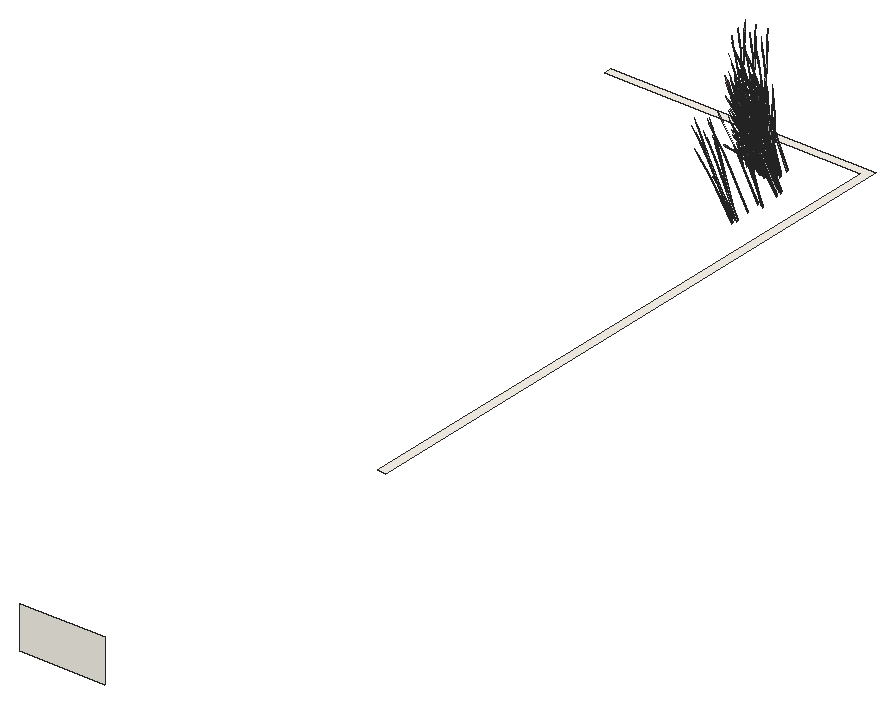
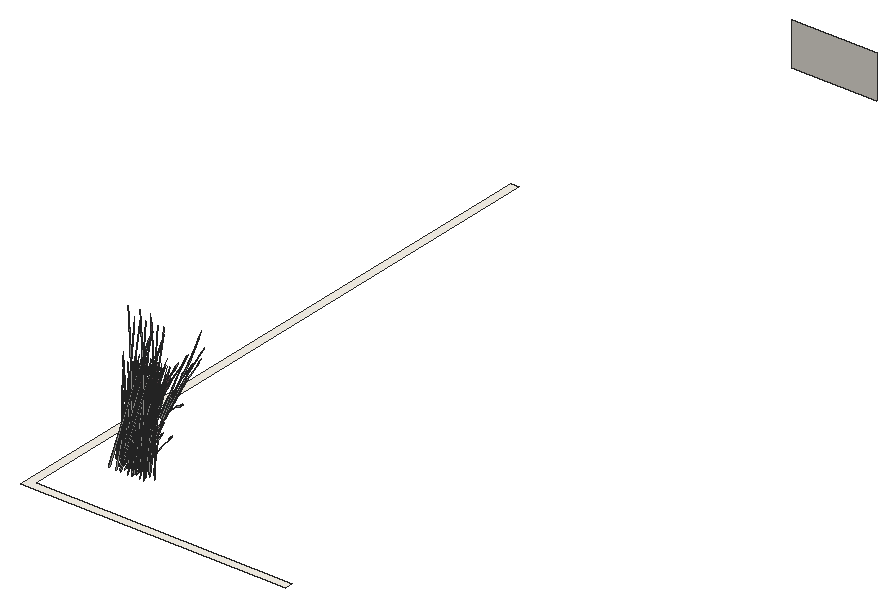
# SketchUp Ruby script. Lengths in inches.
U = 1.inch
M = Sketchup.active_model
def pt(a) = Geom::Point3d.new(a.map { |v| v * U })
def face(e, loops, mat)
  f = e.add_face(loops[0].map { |a| pt(a) })
  loops[1..].each { |l| e.add_face(l.map { |a| pt(a) }).erase! }
  f.material = f.back_material = mat if mat
  f
end
# faces: each face lists its corners as indices into pts; further lists are holes
def faces(e, pts, list, mat = nil) = list.each { |f| face(e, (f[0].is_a?(Array) ? f : [f]).map { |l| l.map { |i| pts[i] } }, mat) }
# xy, xz, yz: faces in a plane at the given z, y or x. An outline is a flat list of corners, or four numbers for a rectangle; further outlines are holes
def ring(l) = l.size == 4 ? [[l[0], l[1]], [l[2], l[1]], [l[2], l[3]], [l[0], l[3]]] : l.each_slice(2).to_a
def flat(e, list, mat, &to3) = list.each { |f| face(e, (f[0].is_a?(Array) ? f : [f]).map { |l| ring(l).map { |u, v| to3.(u, v) } }, mat) }
def xy(e, z, list, mat = nil) = flat(e, list, mat) { |x, y| [x, y, z] }
def xz(e, y, list, mat = nil) = flat(e, list, mat) { |x, z| [x, y, z] }
def yz(e, x, list, mat = nil) = flat(e, list, mat) { |y, z| [x, y, z] }
def lines(e, pts, list) = list.each { |a, b| e.add_line(pt(pts[a]), pt(pts[b])) }
# prism: a flat outline (further loops are holes) pulled along v
def prism(e, loops, v, mat = nil)
  f = face(e, loops, mat); d = Geom::Vector3d.new(v.map { |x| x * U })
  f.pushpull(f.normal.samedirection?(d) ? d.length : -d.length)
end
def box(e, o, s, mat = nil) = prism(e, [[o, [o[0] + s[0], o[1], o[2]], [o[0] + s[0], o[1] + s[1], o[2]], [o[0], o[1] + s[1], o[2]]]], [0, 0, s[2]], mat)
def at(x, y, z, deg = 0) = Geom::Transformation.translation(pt([x, y, z])) * Geom::Transformation.rotation(ORIGIN, Z_AXIS, deg.degrees)
def axes(o, x, y, z) = Geom::Transformation.new([*x, 0, *y, 0, *z, 0, *pt(o).to_a, 1])
def part(name) = M.definitions.add(name)
# library, detail: a bought-in or finely detailed component or shape, given as its bounding box
def library(name, o, s) = part(name).tap { |d| box(d.entities, o, s) }
def detail(e, o, s) = box(e.add_group.entities, o, s)
def put(e, d, t, mat = nil) = e.add_instance(d, t).tap { |i| i.material = mat if mat }
def group(e, t, mat = nil) = e.add_group.tap { |g| g.transformation = t; g.material = mat if mat }.entities
root = M.entities
M.materials.add("C01_Vanilla_Cream").color = [255, 251, 241]
M.materials.add("LightPink_Translucent").color = [144, 107, 117]
M.materials["LightPink_Translucent"].alpha = 0.75
c1 = part("blade")
p = [[2.15,0.21,22],[0,0.17,0],[0.09,0.45,0],[2.18,0.31,22],[2.29,0.31,22],[0.38,0.45,0],
  [2.48,0.24,33],[2.49,0.24,33],[2.48,0.22,33]]
faces(c1.entities,p,[[0,1,2,3],[4,5,2,3],[6,3,4,7],[8,0,3,6]])
c2 = part("seeds")
p = [[0.3,-0.1,1.38],[-0.01,-0.03,1.59],[-0.01,-0.03,0.03],[0.14,-0.07,-0.07],[0.29,-0.03,3],[0.15,0.01,3.11]]
faces(c2.entities,p,[[0,1,2,3],[1,0,4,5]],"LightPink_Translucent")
c3 = part("blade with seeds")
put(c3.entities,c1,at(0,0,0))
put(c3.entities,c2,axes([2.4,0.25,30.99],[1.5799,-0.05474,1.17369],[-0.12525,1.92788,0.29478],[-0.07173,-0.02425,1.56792]))
xy(root,390,[[693.41,144,696.41,144,696.41,360,603,360,603,357,693.41,357]],"C01_Vanilla_Cream")
xz(root,24,[[663.55,375,693.41,390]],"C01_Vanilla_Cream")
put(root,c3,axes([685.68,309.87,392.15],[0.12702,0.15896,1.18691],[-0.2927,0.4321,-0.25526],[-0.30054,-0.10328,0.50747]))
put(root,c3,axes([686.2,309.73,394.13],[-0.65035,-0.01375,-0.58968],[0.04368,-0.5789,0.07116],[-0.27552,-0.06109,0.83415]))
put(root,c3,axes([685.39,310.25,393.22],[0.26985,-0.01293,1.42242],[-0.17902,0.56047,0.11501],[-0.38456,-0.03467,0.60807]))
put(root,c3,axes([686.8,310.65,392.77],[0.18493,-0.0826,1.46963],[0.06377,0.5767,0.11501],[-0.40056,0.07652,0.52526]))
put(root,c3,axes([684.82,311.04,393.91],[-0.10624,0.07413,1.45204],[0.00904,0.54162,-0.22964],[-0.24352,0.07044,0.11645]))
put(root,c3,axes([685.51,311.23,393.22],[0.22574,-0.12077,1.42242],[0.19004,0.55807,0.11501],[-0.35439,0.12613,0.60807]))
put(root,c3,axes([684.8,312.18,392.15],[0.2261,0.04687,1.18691],[0.14573,0.47875,-0.25526],[-0.30712,0.08962,0.50747]))
put(root,c3,axes([686.5625,315.6,393.22],[0.26985,-0.01293,1.42242],[-0.17902,0.56047,0.11501],[-0.38456,-0.03467,0.60807]))
put(root,c3,axes([685.78,320.99,393.22],[0.26985,-0.01293,1.42242],[-0.17902,0.56047,0.11501],[-0.38456,-0.03467,0.60807]))
put(root,c3,axes([687.1875,321.39,392.77],[0.18493,-0.0826,1.46963],[0.06377,0.5767,0.11501],[-0.40056,0.07652,0.52526]))
put(root,c3,axes([685.89,321.98,393.22],[0.22574,-0.12077,1.42242],[0.19004,0.55807,0.11501],[-0.35439,0.12613,0.60807]))
put(root,c3,axes([685.1875,322.93,392.15],[0.2261,0.04687,1.18691],[0.14573,0.47875,-0.25526],[-0.30712,0.08962,0.50747]))
put(root,c3,axes([685.29,329.3,393.22],[0.24166,0.09837,1.42242],[-0.50011,0.41269,0.11501],[-0.3117,-0.18617,0.60807]))
put(root,c3,axes([685.07,329.82,392.15],[0.12702,0.15896,1.18691],[-0.2927,0.4321,-0.25526],[-0.30054,-0.10328,0.50747]))
put(root,c3,axes([685.59,329.68,394.13],[-0.65035,-0.01375,-0.58968],[0.04368,-0.5789,0.07116],[-0.27552,-0.06109,0.83415]))
put(root,c3,axes([685.375,329.8,393.89],[-0.47241,0.37822,-0.42412],[-0.41372,-0.39954,-0.32852],[-0.24002,-0.05755,0.81151]))
put(root,c3,axes([684.78,330.2,393.22],[0.26985,-0.01293,1.42242],[-0.17902,0.56047,0.11501],[-0.38456,-0.03467,0.60807]))
put(root,c3,axes([684.61,330.89,391.24],[0.0165,0.08998,1.46364],[-0.33262,0.46992,-0.2236],[-0.23626,-0.02369,0.24931]))
put(root,c3,axes([684.55,330.6875,393.76],[-0.54068,-0.15928,-0.29394],[0.1577,-0.46469,0.37948],[-0.21769,0.04261,0.72609]))
put(root,c3,axes([686.19,330.61,392.77],[0.18493,-0.0826,1.46963],[0.06377,0.5767,0.11501],[-0.40056,0.07652,0.52526]))
put(root,c3,axes([684.2,330.99,393.91],[-0.10624,0.07413,1.45204],[0.00904,0.54162,-0.22964],[-0.24352,0.07044,0.11645]))
put(root,c3,axes([684.92,330.92,393.89],[-0.17625,0.51936,-0.42412],[-0.60429,-0.17802,-0.32852],[-0.2433,0.04762,0.81151]))
put(root,c3,axes([674.31,337.75,393.22],[0.14872,0.18332,1.42242],[-0.6872,0.15433,0.11501],[-0.15531,-0.28779,0.60807]))
put(root,c3,axes([678.375,337.75,393.22],[0.14872,0.18332,1.42242],[-0.6872,0.15433,0.11501],[-0.15531,-0.28779,0.60807]))
put(root,c3,axes([671.26,336.54,393.91],[-0.09951,-0.08005,1.45204],[-0.66407,0.05075,-0.22964],[-0.10598,-0.19148,0.11645]))
put(root,c3,axes([675.44,336.54,393.91],[-0.09951,-0.08005,1.45204],[-0.66407,0.05075,-0.22964],[-0.10598,-0.19148,0.11645]))
put(root,c3,axes([679.51,336.54,393.91],[-0.09951,-0.08005,1.45204],[-0.66407,0.05075,-0.22964],[-0.10598,-0.19148,0.11645]))
put(root,c3,axes([669.05,337.49,392.15],[-0.18493,0.11557,1.18691],[-0.55384,-0.20228,-0.25526],[0.10266,-0.25157,0.50747]))
put(root,c3,axes([672.8,337.49,392.15],[-0.18493,0.11557,1.18691],[-0.55384,-0.20228,-0.25526],[0.10266,-0.25157,0.50747]))
put(root,c3,axes([676.98,337.49,392.15],[-0.18493,0.11557,1.18691],[-0.55384,-0.20228,-0.25526],[0.10266,-0.25157,0.50747]))
put(root,c3,axes([671.96,337.89,394.13],[-0.31051,-0.46426,-0.58968],[0.63919,-0.25873,0.07116],[-0.07261,-0.22432,0.83415]))
put(root,c3,axes([676.14,337.89,394.13],[-0.31051,-0.46426,-0.58968],[0.63919,-0.25873,0.07116],[-0.07261,-0.22432,0.83415]))
put(root,c3,axes([680.21,337.89,394.13],[-0.31051,-0.46426,-0.58968],[0.63919,-0.25873,0.07116],[-0.07261,-0.22432,0.83415]))
put(root,c3,axes([674.12,337.27,392.15],[-0.0394,0.18678,1.18691],[-0.57594,0.15636,-0.25526],[-0.13463,-0.24142,0.50747]))
put(root,c3,axes([678.1875,337.27,392.15],[-0.0394,0.18678,1.18691],[-0.57594,0.15636,-0.25526],[-0.13463,-0.24142,0.50747]))
put(root,c3,axes([671.42,336.86,391.24],[-0.10912,0.02057,1.46364],[-0.60346,-0.23156,-0.2236],[0.01013,-0.19315,0.24931]))
put(root,c3,axes([675.6,336.86,391.24],[-0.10912,0.02057,1.46364],[-0.60346,-0.23156,-0.2236],[0.01013,-0.19315,0.24931]))
put(root,c3,axes([679.67,336.86,391.24],[-0.10912,0.02057,1.46364],[-0.60346,-0.23156,-0.2236],[0.01013,-0.19315,0.24931]))
put(root,c3,axes([684.9,331.19,393.22],[0.22574,-0.12077,1.42242],[0.19004,0.55807,0.11501],[-0.35439,0.12613,0.60807]))
put(root,c3,axes([669.5,338.35,394.13],[0.01693,-0.52814,-0.58968],[0.71285,0.03547,0.07116],[0.07523,-0.22375,0.83415]))
put(root,c3,axes([673.25,338.35,394.13],[0.01693,-0.52814,-0.58968],[0.71285,0.03547,0.07116],[0.07523,-0.22375,0.83415]))
put(root,c3,axes([677.43,338.35,394.13],[0.01693,-0.52814,-0.58968],[0.71285,0.03547,0.07116],[0.07523,-0.22375,0.83415]))
put(root,c3,axes([670.49,337.52,393.91],[-0.00628,-0.11364,1.45204],[-0.53042,-0.32843,-0.22964],[0.08201,-0.19909,0.11645]))
put(root,c3,axes([674.24,337.52,393.91],[-0.00628,-0.11364,1.45204],[-0.53042,-0.32843,-0.22964],[0.08201,-0.19909,0.11645]))
put(root,c3,axes([678.43,337.52,393.91],[-0.00628,-0.11364,1.45204],[-0.53042,-0.32843,-0.22964],[0.08201,-0.19909,0.11645]))
put(root,c3,axes([672.02,337.5,393.76],[0.19614,-0.43908,-0.29394],[0.57222,0.12807,0.37948],[-0.05247,-0.17678,0.72609]))
put(root,c3,axes([676.2,337.5,393.76],[0.19614,-0.43908,-0.29394],[0.57222,0.12807,0.37948],[-0.05247,-0.17678,0.72609]))
put(root,c3,axes([680.27,337.5,393.76],[0.19614,-0.43908,-0.29394],[0.57222,0.12807,0.37948],[-0.05247,-0.17678,0.72609]))
put(root,c3,axes([668.7,338.08,393.22],[-0.12114,0.19625,1.42242],[-0.50818,-0.40613,0.11501],[0.22925,-0.25313,0.60807]))
put(root,c3,axes([672.45,338.08,393.22],[-0.12114,0.19625,1.42242],[-0.50818,-0.40613,0.11501],[0.22925,-0.25313,0.60807]))
put(root,c3,axes([670.35,337.11,393.91],[-0.06607,0.04361,1.47228],[-0.64734,-0.14714,-0.13912],[-0.02343,-0.19032,0.26054]))
put(root,c3,axes([674.1,337.11,393.91],[-0.06607,0.04361,1.47228],[-0.64734,-0.14714,-0.13912],[-0.02343,-0.19032,0.26054]))
put(root,c3,axes([678.28,337.11,393.91],[-0.06607,0.04361,1.47228],[-0.64734,-0.14714,-0.13912],[-0.02343,-0.19032,0.26054]))
put(root,c3,axes([671.72,337.8,393.89],[-0.63954,-0.14313,-0.42412],[0.21921,-0.49074,-0.32852],[-0.05864,-0.19758,0.81151]))
put(root,c3,axes([675.91,337.8,393.89],[-0.63954,-0.14313,-0.42412],[0.21921,-0.49074,-0.32852],[-0.05864,-0.19758,0.81151]))
put(root,c3,axes([679.97,337.8,393.89],[-0.63954,-0.14313,-0.42412],[0.21921,-0.49074,-0.32852],[-0.05864,-0.19758,0.81151]))
put(root,c3,axes([668.37,336.57,392.3],[0.08346,0.33295,0.95334],[-0.46298,-0.1844,0.70045],[0.04982,-0.17048,0.20998]))
put(root,c3,axes([672.12,336.57,392.3],[0.08346,0.33295,0.95334],[-0.46298,-0.1844,0.70045],[0.04982,-0.17048,0.20998]))
put(root,c3,axes([676.3,336.57,392.3],[0.08346,0.33295,0.95334],[-0.46298,-0.1844,0.70045],[0.04982,-0.17048,0.20998]))
put(root,c3,axes([684.19,332.14,392.15],[0.2261,0.04687,1.18691],[0.14573,0.47875,-0.25526],[-0.30712,0.08962,0.50747]))
put(root,c3,axes([669.36,338.17,393.89],[-0.46573,-0.38364,-0.42412],[0.49199,-0.33598,-0.32852],[0.07086,-0.19492,0.81151]))
put(root,c3,axes([673.11,338.17,393.89],[-0.46573,-0.38364,-0.42412],[0.49199,-0.33598,-0.32852],[0.07086,-0.19492,0.81151]))
put(root,c3,axes([677.29,338.17,393.89],[-0.46573,-0.38364,-0.42412],[0.49199,-0.33598,-0.32852],[0.07086,-0.19492,0.81151]))
put(root,c3,axes([683.02,331.54,393.91],[0.08303,0.01531,1.47228],[0.25685,0.50448,-0.13912],[-0.16996,0.13241,0.26054]))
put(root,c3,axes([674.76,336.28,393.91],[-0.01214,0.06844,1.47228],[-0.59861,0.24837,-0.13912],[-0.17615,-0.12696,0.26054]))
put(root,c3,axes([678.83,336.28,393.91],[-0.01214,0.06844,1.47228],[-0.59861,0.24837,-0.13912],[-0.17615,-0.12696,0.26054]))
put(root,c3,axes([674.63,337.49,394.23],[0.72473,-0.14676,0.44623],[0.12578,0.57568,0.36794],[-0.17045,-0.16967,0.92337]))
put(root,c3,axes([678.7,337.49,394.23],[0.72473,-0.14676,0.44623],[0.12578,0.57568,0.36794],[-0.17045,-0.16967,0.92337]))
put(root,c3,axes([672.09,337.6,393.93],[0.64106,0.14927,0.39842],[-0.21921,0.49074,0.32852],[-0.03852,-0.19299,0.82444]))
put(root,c3,axes([676.27,337.6,393.93],[0.64106,0.14927,0.39842],[-0.21921,0.49074,0.32852],[-0.03852,-0.19299,0.82444]))
put(root,c3,axes([672.27,337.77,394.18],[-0.63664,0.26583,-0.10093],[-0.31286,-0.47181,-0.56021],[-0.084,-0.19882,0.85122]))
put(root,c3,axes([676.45,337.77,394.18],[-0.63664,0.26583,-0.10093],[-0.31286,-0.47181,-0.56021],[-0.084,-0.19882,0.85122]))
put(root,c3,axes([680.52,337.77,394.18],[-0.63664,0.26583,-0.10093],[-0.31286,-0.47181,-0.56021],[-0.084,-0.19882,0.85122]))
put(root,c3,axes([669.84,338.37,394.18],[-0.71502,-0.02829,-0.10093],[0.01954,-0.53563,-0.56021],[0.04967,-0.20629,0.85122]))
put(root,c3,axes([673.59,338.37,394.18],[-0.71502,-0.02829,-0.10093],[0.01954,-0.53563,-0.56021],[0.04967,-0.20629,0.85122]))
put(root,c3,axes([677.78,338.37,394.18],[-0.71502,-0.02829,-0.10093],[0.01954,-0.53563,-0.56021],[0.04967,-0.20629,0.85122]))
put(root,c3,axes([669.79,338.03,393.76],[0.4402,-0.30062,-0.29394],[0.41671,0.34326,0.37948],[0.0634,-0.1744,0.72609]))
put(root,c3,axes([673.54,338.03,393.76],[0.4402,-0.30062,-0.29394],[0.41671,0.34326,0.37948],[0.0634,-0.1744,0.72609]))
put(root,c3,axes([677.73,338.03,393.76],[0.4402,-0.30062,-0.29394],[0.41671,0.34326,0.37948],[0.0634,-0.1744,0.72609]))
put(root,c3,axes([673.92,336.97,392.3],[0.33937,0.19872,0.95334],[-0.49424,0.11946,0.70045],[-0.10575,-0.15273,0.20998]))
put(root,c3,axes([677.99,336.97,392.3],[0.33937,0.19872,0.95334],[-0.49424,0.11946,0.70045],[-0.10575,-0.15273,0.20998]))
put(root,c3,axes([672.26,337.5625,393.93],[0.47939,-0.19405,0.05337],[0.23464,0.35385,0.42015],[-0.0463,-0.15598,0.64067]))
put(root,c3,axes([676.4375,337.5625,393.93],[0.47939,-0.19405,0.05337],[0.23464,0.35385,0.42015],[-0.0463,-0.15598,0.64067]))
put(root,c3,axes([680.51,337.5625,393.93],[0.47939,-0.19405,0.05337],[0.23464,0.35385,0.42015],[-0.0463,-0.15598,0.64067]))
put(root,c3,axes([674.74,338.02,394.13],[-0.55475,-0.27598,-0.58968],[0.39425,-0.48361,0.07116],[-0.20099,-0.16478,0.83415]))
put(root,c3,axes([678.81,338.02,394.13],[-0.55475,-0.27598,-0.58968],[0.39425,-0.48361,0.07116],[-0.20099,-0.16478,0.83415]))
put(root,c3,axes([674.55,337.66,393.76],[-0.10048,-0.4599,-0.29394],[0.5744,-0.12144,0.37948],[-0.15428,-0.13179,0.72609]))
put(root,c3,axes([678.62,337.66,393.76],[-0.10048,-0.4599,-0.29394],[0.5744,-0.12144,0.37948],[-0.15428,-0.13179,0.72609]))
put(root,c3,axes([674.8,337.62,393.93],[0.29569,-0.36271,0.05337],[0.42107,0.21117,0.42015],[-0.13613,-0.11629,0.64067]))
put(root,c3,axes([678.87,337.62,393.93],[0.29569,-0.36271,0.05337],[0.42107,0.21117,0.42015],[-0.13613,-0.11629,0.64067]))
put(root,c3,axes([673.65,337.57,391.24],[-0.06302,0.07522,1.46364],[-0.63686,0.16217,-0.2236],[-0.15385,-0.14752,0.24931]))
put(root,c3,axes([677.72,337.57,391.24],[-0.06302,0.07522,1.46364],[-0.63686,0.16217,-0.2236],[-0.15385,-0.14752,0.24931]))
put(root,c3,axes([670.52,339.64,391.74],[-0.26718,-0.5855,-0.57963],[0.76964,-0.21087,-0.15213],[-0.02953,-0.19827,1.27944]))
put(root,c3,axes([674.7,339.64,391.74],[-0.26718,-0.5855,-0.57963],[0.76964,-0.21087,-0.15213],[-0.02953,-0.19827,1.27944]))
put(root,c3,axes([678.77,339.64,391.74],[-0.26718,-0.5855,-0.57963],[0.76964,-0.21087,-0.15213],[-0.02953,-0.19827,1.27944]))
put(root,c3,axes([677.38,338.33,393.22],[0.24166,0.09837,1.42242],[-0.50011,0.41269,0.11501],[-0.3117,-0.18617,0.60807]))
put(root,c3,axes([670.34,337.85,391.24],[-0.09738,-0.04498,1.46364],[-0.25012,-0.50252,-0.2236],[0.16873,-0.13637,0.24931]))
put(root,c3,axes([674.09,337.85,391.24],[-0.09738,-0.04498,1.46364],[-0.25012,-0.50252,-0.2236],[0.16873,-0.13637,0.24931]))
put(root,c3,axes([672.08,337.96,394.19],[-0.19614,0.43908,0.29394],[-0.57222,-0.12807,-0.37948],[-0.05247,-0.17678,0.72609]))
put(root,c3,axes([676.26,337.96,394.19],[-0.19614,0.43908,0.29394],[-0.57222,-0.12807,-0.37948],[-0.05247,-0.17678,0.72609]))
put(root,c3,axes([680.33,337.96,394.19],[-0.19614,0.43908,0.29394],[-0.57222,-0.12807,-0.37948],[-0.05247,-0.17678,0.72609]))
put(root,c3,axes([674.48,338.04,393.89],[-0.64198,0.13573,-0.42412],[-0.1123,-0.514,-0.32852],[-0.17243,-0.1473,0.81151]))
put(root,c3,axes([678.55,338.04,393.89],[-0.64198,0.13573,-0.42412],[-0.1123,-0.514,-0.32852],[-0.17243,-0.1473,0.81151]))
put(root,c3,axes([669.79,338.14,393.93],[0.46327,0.38957,0.39842],[-0.49199,0.33598,0.32852],[0.08546,-0.18277,0.82444]))
put(root,c3,axes([673.54,338.14,393.93],[0.46327,0.38957,0.39842],[-0.49199,0.33598,0.32852],[0.08546,-0.18277,0.82444]))
put(root,c3,axes([677.72,338.14,393.93],[0.46327,0.38957,0.39842],[-0.49199,0.33598,0.32852],[0.08546,-0.18277,0.82444]))
put(root,c3,axes([674.93,337.58,394.51],[-0.4342,0.54737,-0.11304],[-0.6288,-0.31535,-0.62743],[-0.21858,-0.15465,0.95337]))
put(root,c3,axes([679,337.58,394.51],[-0.4342,0.54737,-0.11304],[-0.6288,-0.31535,-0.62743],[-0.21858,-0.15465,0.95337]))
put(root,c3,axes([669.96,338.18,393.93],[0.53464,0.0266,0.05337],[-0.01466,0.40172,0.42015],[0.05594,-0.15388,0.64067]))
put(root,c3,axes([673.71,338.18,393.93],[0.53464,0.0266,0.05337],[-0.01466,0.40172,0.42015],[0.05594,-0.15388,0.64067]))
put(root,c3,axes([677.89,338.18,393.93],[0.53464,0.0266,0.05337],[-0.01466,0.40172,0.42015],[0.05594,-0.15388,0.64067]))
put(root,c3,axes([669.5625,338.45,394.19],[-0.4402,0.30062,0.29394],[-0.41671,-0.34326,-0.37948],[0.0634,-0.1744,0.72609]))
put(root,c3,axes([673.3125,338.45,394.19],[-0.4402,0.30062,0.29394],[-0.41671,-0.34326,-0.37948],[0.0634,-0.1744,0.72609]))
put(root,c3,axes([677.5,338.45,394.19],[-0.4402,0.30062,0.29394],[-0.41671,-0.34326,-0.37948],[0.0634,-0.1744,0.72609]))
put(root,c3,axes([670.34,339.26,394.13],[0.33983,-0.45051,-0.58968],[0.59551,0.32017,0.07116],[0.20291,-0.16322,0.83415]))
put(root,c3,axes([674.09,339.26,394.13],[0.33983,-0.45051,-0.58968],[0.59551,0.32017,0.07116],[0.20291,-0.16322,0.83415]))
put(root,c3,axes([666.67,337.95,391.97],[-0.40676,-0.57214,0],[0.68052,-0.31907,-0.42834],[0.15499,-0.07267,1.3588]))
put(root,c3,axes([670.42,337.95,391.97],[-0.40676,-0.57214,0],[0.68052,-0.31907,-0.42834],[0.15499,-0.07267,1.3588]))
put(root,c3,axes([674.6,337.95,391.97],[-0.40676,-0.57214,0],[0.68052,-0.31907,-0.42834],[0.15499,-0.07267,1.3588]))
put(root,c3,axes([670.32,339.05,393.89],[-0.16713,-0.52135,-0.42412],[0.63294,-0.0912,-0.32852],[0.18138,-0.14003,0.81151]))
put(root,c3,axes([674.07,339.05,393.89],[-0.16713,-0.52135,-0.42412],[0.63294,-0.0912,-0.32852],[0.18138,-0.14003,0.81151]))
put(root,c3,axes([671.31,337.26,391.77],[-0.44958,0.32756,-0.03231],[-0.41194,-0.35875,-0.14649],[-0.029,-0.10165,0.48318]))
put(root,c3,axes([675.49,337.26,391.77],[-0.44958,0.32756,-0.03231],[-0.41194,-0.35875,-0.14649],[-0.029,-0.10165,0.48318]))
put(root,c3,axes([679.56,337.26,391.77],[-0.44958,0.32756,-0.03231],[-0.41194,-0.35875,-0.14649],[-0.029,-0.10165,0.48318]))
put(root,c3,axes([677.33,337.42,393.91],[-0.13998,-0.00403,1.45204],[-0.44565,0.40302,-0.22964],[-0.23779,-0.08235,0.11645]))
put(root,c3,axes([670.62,339.43,394.18],[-0.60181,-0.31483,-0.10093],[0.34671,-0.45593,-0.56021],[0.17003,-0.15849,0.85122]))
put(root,c3,axes([674.37,339.43,394.18],[-0.60181,-0.31483,-0.10093],[0.34671,-0.45593,-0.56021],[0.17003,-0.15849,0.85122]))
put(root,c3,axes([676.07,341.15,392.76],[0.56221,0.23024,1.25546],[-0.55078,0.49601,0.49647],[-0.2467,-0.29398,1.05249]))
put(root,c3,axes([680.14,341.15,392.76],[0.56221,0.23024,1.25546],[-0.55078,0.49601,0.49647],[-0.2467,-0.29398,1.05249]))
put(root,c3,axes([674.89,338.03,394.19],[0.10048,0.4599,0.29394],[-0.5744,0.12144,-0.37948],[-0.15428,-0.13179,0.72609]))
put(root,c3,axes([678.96,338.03,394.19],[0.10048,0.4599,0.29394],[-0.5744,0.12144,-0.37948],[-0.15428,-0.13179,0.72609]))
put(root,c3,axes([668.95,339.55,391.67],[0,-0.57097,-0.4121],[0.72788,0,0],[0,-0.13004,1.30728]))
put(root,c3,axes([673.13,339.55,391.67],[0,-0.57097,-0.4121],[0.72788,0,0],[0,-0.13004,1.30728]))
put(root,c3,axes([677.2,339.55,391.67],[0,-0.57097,-0.4121],[0.72788,0,0],[0,-0.13004,1.30728]))
